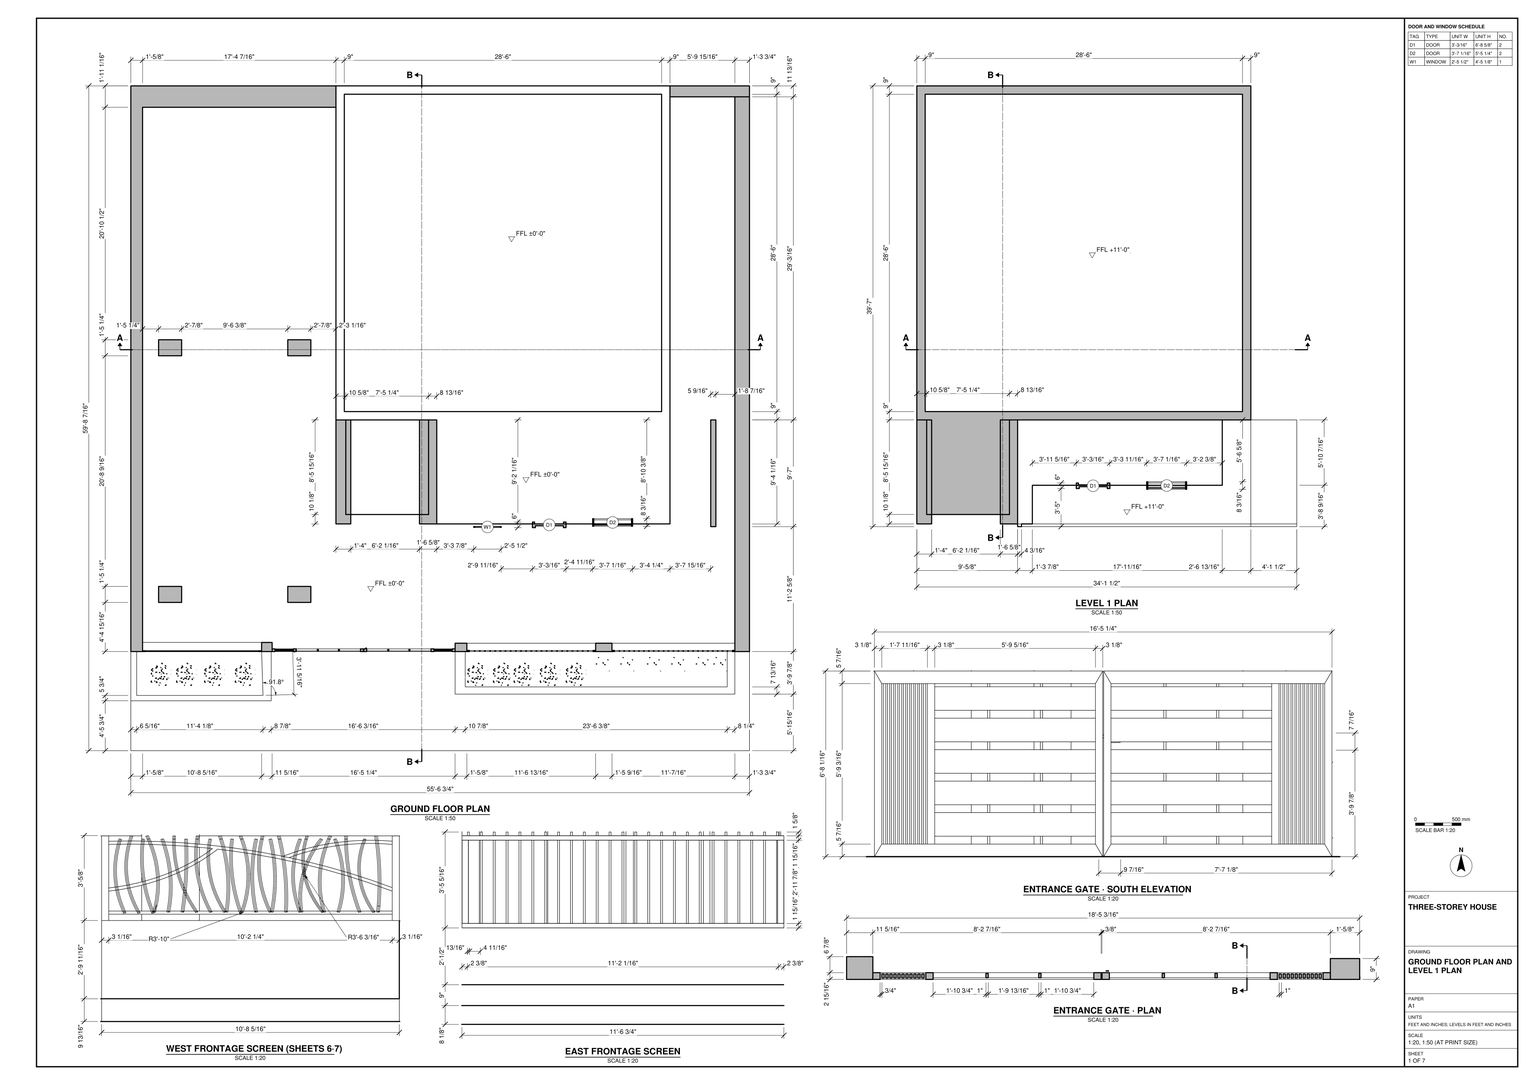
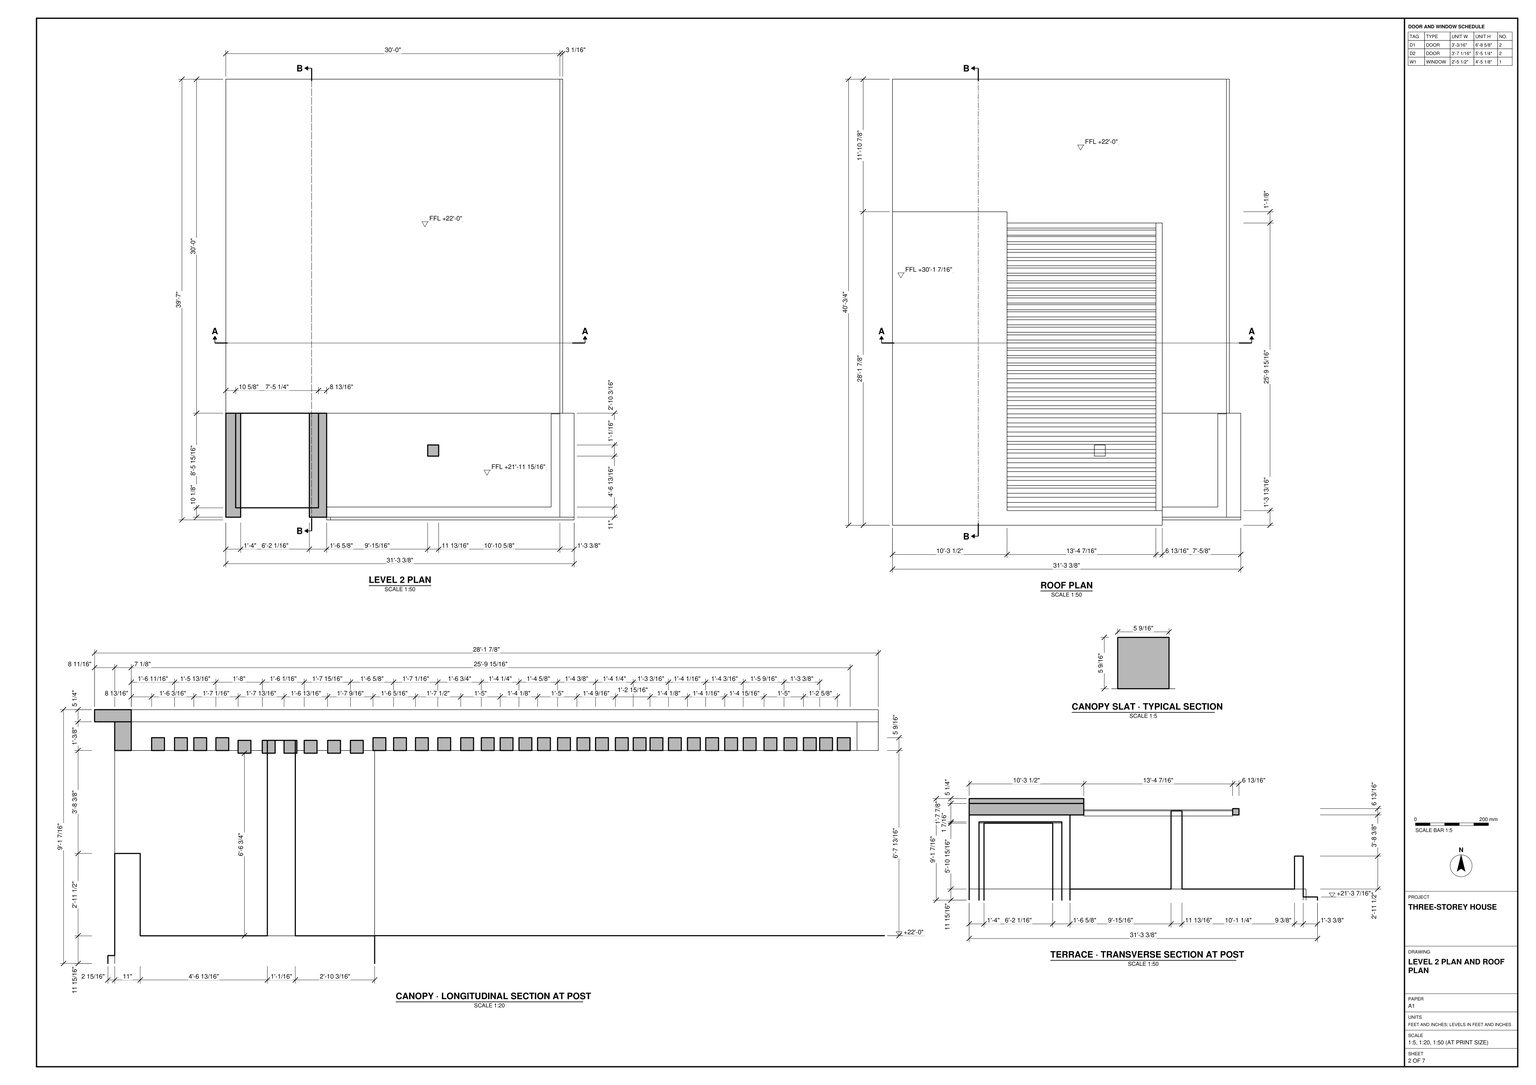
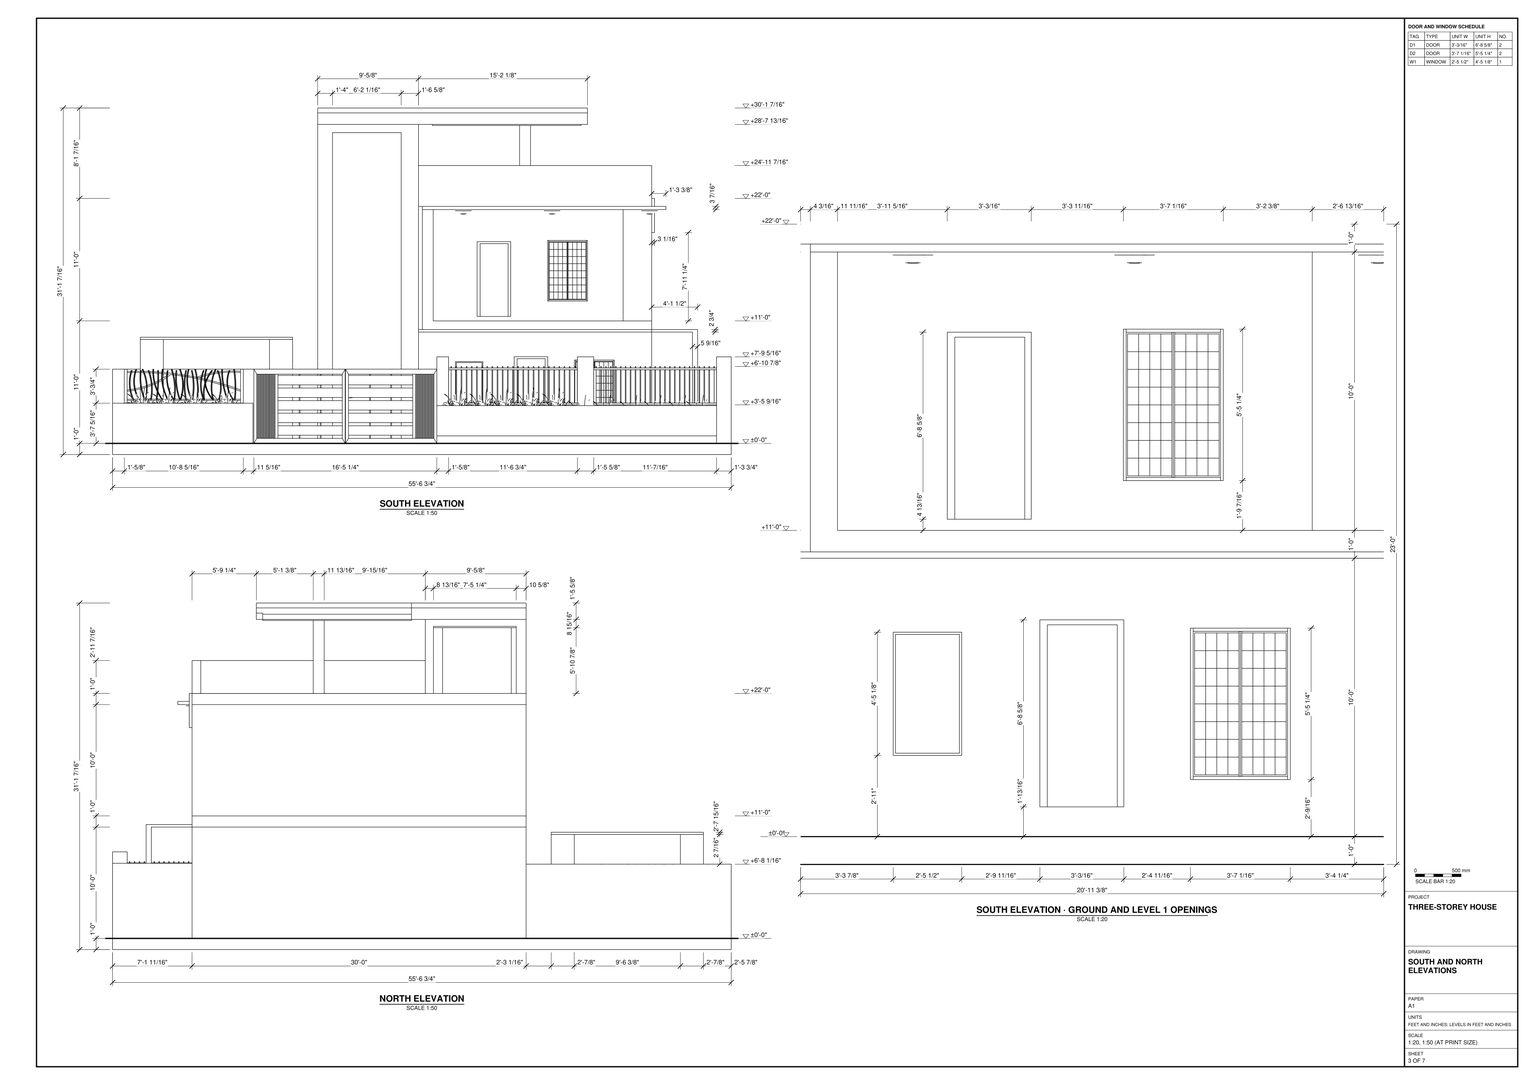
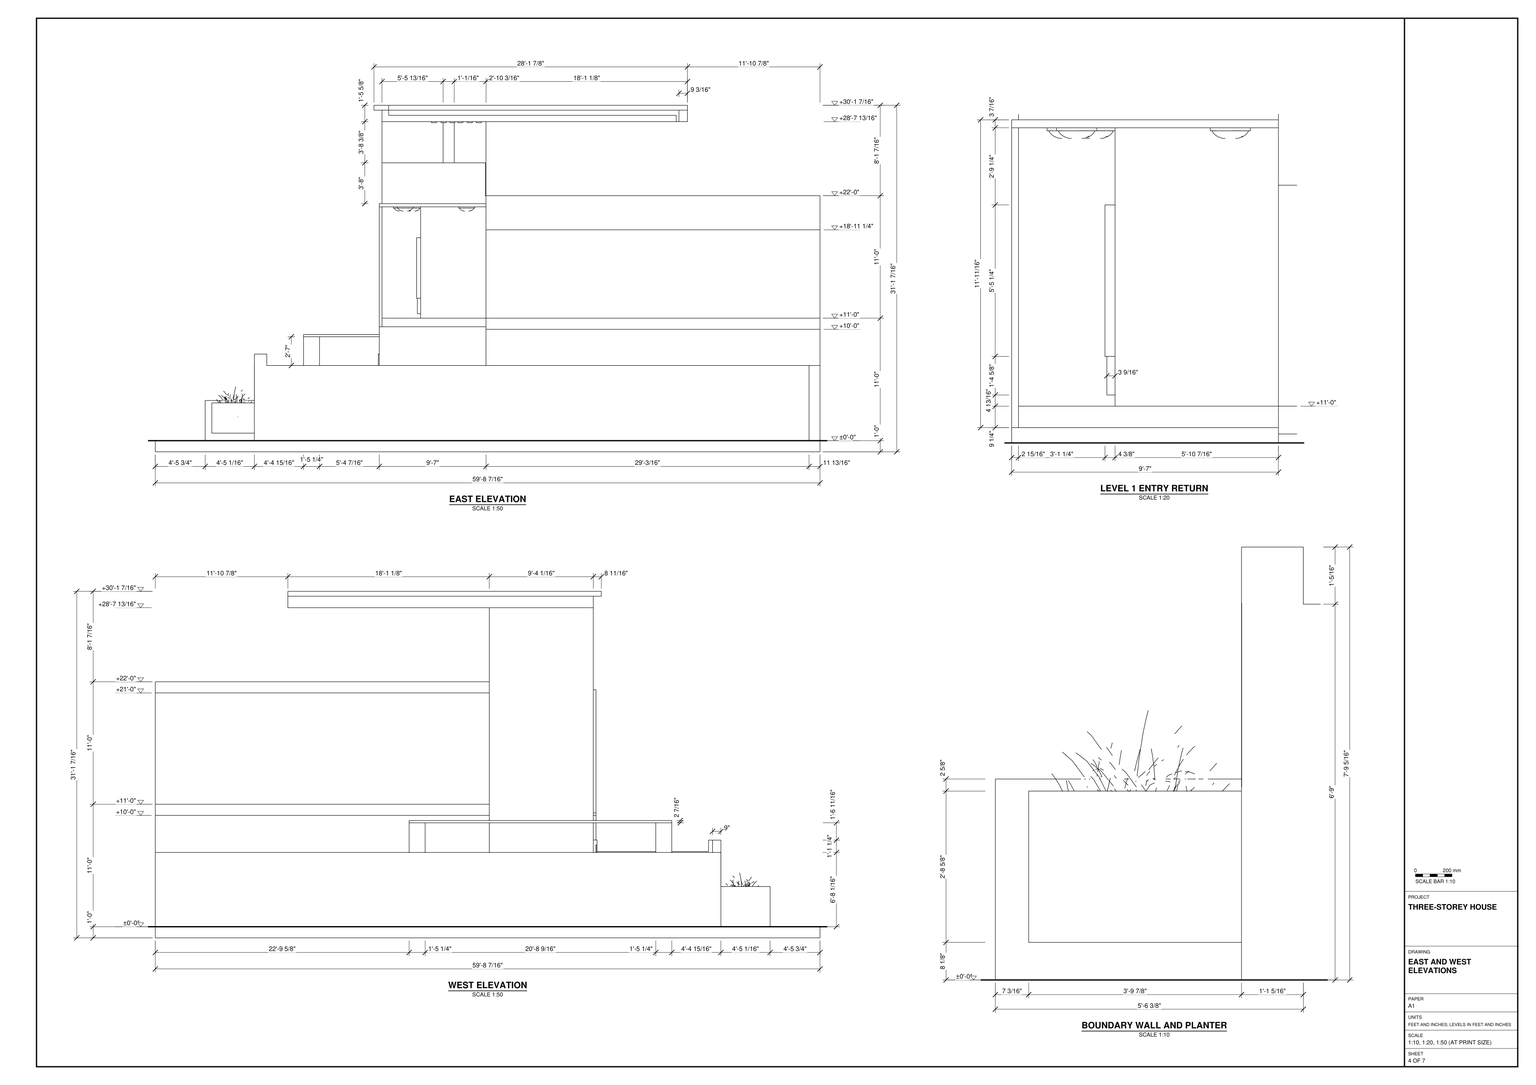
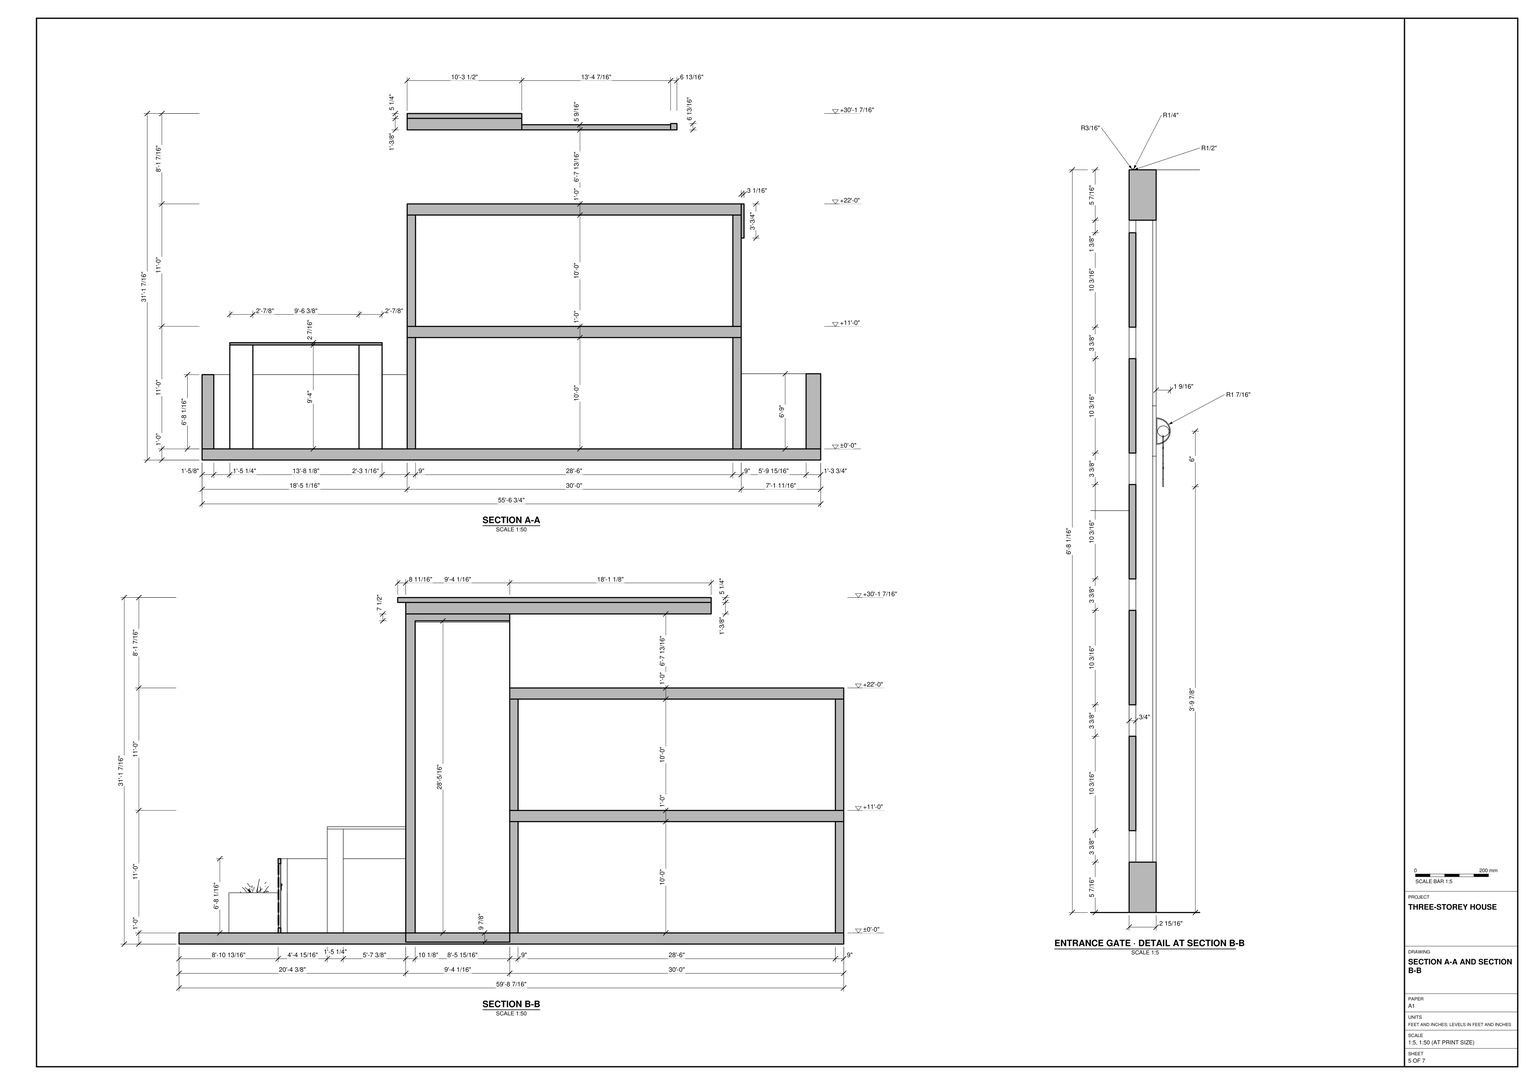
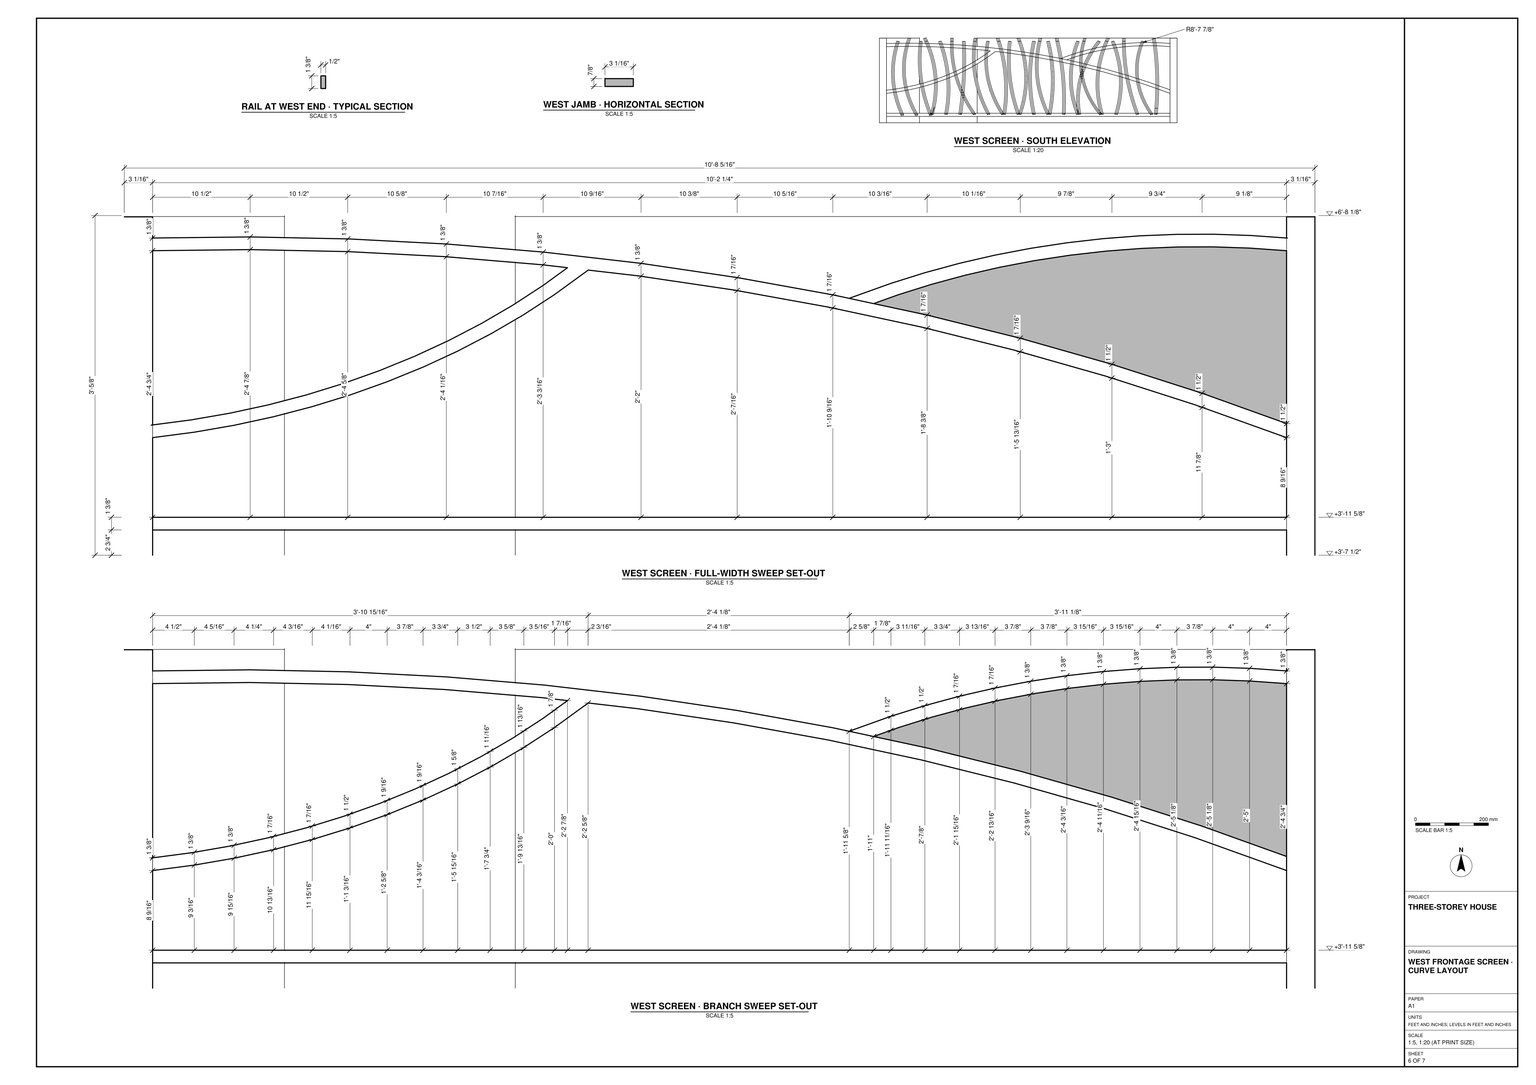
Work in feet and inches in SketchUp, using the plans, elevations, sections and details in task_files/diagram_01.pdf. Model the house and its enclosed site. The overall model measures 55'-6 3/4" east to west, 59'-8 7/16" north to south and 31'-1 7/16" high. Set the ground floor at ±0'-0", the next floor at +11'-0" and the terrace level at +22'-0".

Place the main block toward the rear of the site, leaving the forecourt between the house and the south entrance. Follow the wall thicknesses on the plans, including the 9" walls of the main block. Use the sections and elevations to set the slab edges, recesses and projections. Fit the doors, grilles and window in the south walls at the positions and heights shown. Above them, model the terrace parapet and the canopy, distinguishing its solid roof strip from the open span of parallel slats on posts.

Continue the site walls to the south frontage. Model the paired entrance gate, the curved-bar screen to its west, the vertical-bar screens to its east and the planting beds flanking the entrance. Decor and loose items, including plants, may be any suitable library components. Keep shell elements and individual furniture or joinery pieces in separate groups or components, and use components for repeated parts. Save one SketchUp model as output_files/three_storey_house_screened_frontage_and_terrace_canopy.skp.

# SketchUp Ruby script. Lengths in inches.
U = 1.inch
M = Sketchup.active_model
def pt(a) = Geom::Point3d.new(a.map { |v| v * U })
def face(e, loops, mat)
  f = e.add_face(loops[0].map { |a| pt(a) })
  loops[1..].each { |l| e.add_face(l.map { |a| pt(a) }).erase! }
  f.material = f.back_material = mat if mat
  f
end
# faces: each face lists its corners as indices into pts; further lists are holes
def faces(e, pts, list, mat = nil) = list.each { |f| face(e, (f[0].is_a?(Array) ? f : [f]).map { |l| l.map { |i| pts[i] } }, mat) }
# xy, xz, yz: faces in a plane at the given z, y or x. An outline is a flat list of corners, or four numbers for a rectangle; further outlines are holes
def ring(l) = l.size == 4 ? [[l[0], l[1]], [l[2], l[1]], [l[2], l[3]], [l[0], l[3]]] : l.each_slice(2).to_a
def flat(e, list, mat, &to3) = list.each { |f| face(e, (f[0].is_a?(Array) ? f : [f]).map { |l| ring(l).map { |u, v| to3.(u, v) } }, mat) }
def xy(e, z, list, mat = nil) = flat(e, list, mat) { |x, y| [x, y, z] }
def xz(e, y, list, mat = nil) = flat(e, list, mat) { |x, z| [x, y, z] }
def yz(e, x, list, mat = nil) = flat(e, list, mat) { |y, z| [x, y, z] }
def lines(e, pts, list) = list.each { |a, b| e.add_line(pt(pts[a]), pt(pts[b])) }
# prism: a flat outline (further loops are holes) pulled along v
def prism(e, loops, v, mat = nil)
  f = face(e, loops, mat); d = Geom::Vector3d.new(v.map { |x| x * U })
  f.pushpull(f.normal.samedirection?(d) ? d.length : -d.length)
end
def box(e, o, s, mat = nil) = prism(e, [[o, [o[0] + s[0], o[1], o[2]], [o[0] + s[0], o[1] + s[1], o[2]], [o[0], o[1] + s[1], o[2]]]], [0, 0, s[2]], mat)
def at(x, y, z, deg = 0) = Geom::Transformation.translation(pt([x, y, z])) * Geom::Transformation.rotation(ORIGIN, Z_AXIS, deg.degrees)
def axes(o, x, y, z) = Geom::Transformation.new([*x, 0, *y, 0, *z, 0, *pt(o).to_a, 1])
def part(name) = M.definitions.add(name)
# library, detail: a bought-in or finely detailed component or shape, given as its bounding box
def library(name, o, s) = part(name).tap { |d| box(d.entities, o, s) }
def detail(e, o, s) = box(e.add_group.entities, o, s)
def put(e, d, t, mat = nil) = e.add_instance(d, t).tap { |i| i.material = mat if mat }
def group(e, t, mat = nil) = e.add_group.tap { |g| g.transformation = t; g.material = mat if mat }.entities
root = M.entities
M.materials.add("Shane").color = [124, 51, 43]
M.materials.add("[Color M00]").color = [255, 255, 255]
M.materials.add("[Color M07]").color = [58, 58, 58]
M.materials.add("[Color M08]").color = [30, 30, 30]
M.materials.add("[Gray4]").color = [170, 170, 170]
M.materials.add("[Gray8]").color = [68, 68, 68]
M.materials.add("[Slate]").color = [102, 110, 108]
M.materials.add("[Translucent Glass Gray]3").color = [128, 128, 128]
M.materials["[Translucent Glass Gray]3"].alpha = 0.3
M.materials.add("[Translucent_Glass_Gray]").color = [128, 128, 128]
M.materials["[Translucent_Glass_Gray]"].alpha = 0.5
M.materials.add("[Wood Floor Light]").color = [204, 176, 127]
M.materials.add("[Wood Floor]").color = [155, 105, 61]
M.materials.add("[Wood_Cherry_Original]").color = [152, 86, 42]
c1 = part("door 15\#1")
xy(c1.entities,0,[[0,0,0,6,2.34,6,2.34,4,33.41,4,33.41,6,36.21,6,36.21,0,33.4,0,33.4,2,3.22,2,3.22,0]],"Shane")
xy(c1.entities,78.49,[[3.22,0,33.4,2]],"Shane")
xy(c1.entities,78.6875,[[2.34,4,33.41,6]],"Shane")
xy(c1.entities,80.63,[[0,0,36.21,6]],"Shane")
xz(c1.entities,0,[[0,0,3.22,0,3.22,78.49,33.4,78.49,33.4,0,36.21,0,36.21,80.63,0,80.63]],"Shane")
xz(c1.entities,2,[[3.22,0,33.4,78.49]],"Shane")
xz(c1.entities,4,[[2.34,0,33.41,78.6875]],"Shane")
xz(c1.entities,6,[[0,0,0,80.63,36.21,80.63,36.21,0,33.41,0,33.41,78.6875,2.34,78.6875,2.34,0]],"Shane")
yz(c1.entities,0,[[0,0,6,80.63]],"Shane")
yz(c1.entities,2.34,[[4,0,6,78.6875]],"Shane")
yz(c1.entities,3.22,[[0,0,2,78.49]],"Shane")
yz(c1.entities,33.4,[[0,0,2,78.49]],"Shane")
yz(c1.entities,33.41,[[4,0,6,78.6875]],"Shane")
yz(c1.entities,36.21,[[0,0,6,80.63]],"Shane")
c2 = part("glass door")
xy(c2.entities,0,[[0,-12,72,0]],"[Wood_Cherry_Original]")
xy(c2.entities,2,[[35,-10,36,-8],[36,-10,37,-8]],"[Gray4]")
xy(c2.entities,2,[[2,-10,35,-8],[37,-10,70,-8]],"[Gray8]")
xy(c2.entities,2,[[2,-12,70,-10],[2,-8,70,-2],[2,-2,70,0]],"[Wood_Cherry_Original]")
xy(c2.entities,94,[[35,-10,36,-8],[36,-10,37,-8]],"[Gray4]")
xy(c2.entities,94,[[2,-10,35,-8],[37,-10,70,-8]],"[Gray8]")
xy(c2.entities,94,[[2,-12,70,-10],[2,-8,70,0]],"[Wood_Cherry_Original]")
xy(c2.entities,96,[[0,-12,2,0],[2,-12,70,0],[70,-12,72,0]],"[Wood_Cherry_Original]")
xz(c2.entities,-12,[[0,0,2,96],[2,0,70,2],[70,0,72,96],[2,94,70,96]],"[Wood_Cherry_Original]")
xz(c2.entities,-10,[[3,3,11,14.25],[11,3,19,14.25],[19,3,27,14.25],[27,3,35,14.25],[37,3,45,14.25],
  [45,3,53,14.25],[53,3,61,14.25],[61,3,69,14.25],[3,14.25,11,25.5],[11,14.25,19,25.5],
  [19,14.25,27,25.5],[27,14.25,35,25.5],[37,14.25,45,25.5],[45,14.25,53,25.5],[53,14.25,61,25.5],
  [61,14.25,69,25.5],[3,25.5,11,36.75],[11,25.5,19,36.75],[19,25.5,27,36.75],[27,25.5,35,36.75],
  [37,25.5,45,36.75],[45,25.5,53,36.75],[53,25.5,61,36.75],[61,25.5,69,36.75],[3,36.75,11,48],
  [11,36.75,19,48],[19,36.75,27,48],[27,36.75,35,48],[37,36.75,45,48],[45,36.75,53,48],
  [53,36.75,61,48],[61,36.75,69,48],[3,48,11,59.25],[11,48,19,59.25],[19,48,27,59.25],
  [27,48,35,59.25],[37,48,45,59.25],[45,48,53,59.25],[53,48,61,59.25],[61,48,69,59.25],
  [3,59.25,11,70.5],[11,59.25,19,70.5],[19,59.25,27,70.5],[27,59.25,35,70.5],[37,59.25,45,70.5],
  [45,59.25,53,70.5],[53,59.25,61,70.5],[61,59.25,69,70.5],[3,70.5,11,81.75],[11,70.5,19,81.75],
  [19,70.5,27,81.75],[27,70.5,35,81.75],[37,70.5,45,81.75],[45,70.5,53,81.75],[53,70.5,61,81.75],
  [61,70.5,69,81.75],[3,81.75,11,93],[11,81.75,19,93],[19,81.75,27,93],[27,81.75,35,93],
  [37,81.75,45,93],[45,81.75,53,93],[53,81.75,61,93],[61,81.75,69,93]],"[Translucent_Glass_Gray]")
xz(c2.entities,-10,[[2,2,2,94,35,94,35,93,3,93,3,3,35,3,35,2],[35,2,36,94],[36,2,37,94],[37,2,37,3,69,3,69,93,37,93,37,94,70,94,70,2]],"[Wood_Cherry_Original]")
xz(c2.entities,0,[[0,0,72,0,72,96,70,96,70,2,2,2,2,96,0,96],[2,94,70,96]],"[Wood_Cherry_Original]")
yz(c2.entities,0,[[-12,0,0,96]],"[Wood_Cherry_Original]")
yz(c2.entities,2,[[-12,94,-10,96],[-10,94,-8,96],[-8,94,-2,96],[-2,94,0,96]])
yz(c2.entities,2,[[-10,2,-8,94]],"[Gray8]")
yz(c2.entities,2,[[-12,2,-10,94],[-8,2,-2,94],[-2,2,0,94]],"[Wood_Cherry_Original]")
yz(c2.entities,70,[[-12,94,-10,96],[-10,94,-8,96],[-8,94,-2,96],[-2,94,0,96]])
yz(c2.entities,70,[[-10,2,-8,94]],"[Gray8]")
yz(c2.entities,70,[[-12,2,-10,94],[-8,2,-2,94],[-2,2,0,94]],"[Wood_Cherry_Original]")
yz(c2.entities,72,[[-12,0,0,96]],"[Wood_Cherry_Original]")
c3 = part("WINDOW")
xy(c3.entities,0,[[0,0,59.06,1.97]],"[Color M07]")
xy(c3.entities,1.97,[[1.97,0,57.09,0.98],[1.97,0.98,57.09,1.97]],"[Color M07]")
xy(c3.entities,104.33,[[1.97,0,57.09,0.98],[1.97,0.98,57.09,1.97]],"[Color M07]")
xy(c3.entities,106.3,[[0,0,59.06,1.97]],"[Color M07]")
xz(c3.entities,0,[[[0,0,59.06,106.3],[1.97,1.97,57.09,104.33]]],"[Color M07]")
xz(c3.entities,0.98,[[1.97,1.97,57.09,104.33]],"[Translucent Glass Gray]3")
xz(c3.entities,1.97,[[[0,0,59.06,106.3],[1.97,1.97,57.09,104.33]]],"[Color M07]")
yz(c3.entities,0,[[0,0,1.97,106.3]],"[Color M07]")
yz(c3.entities,1.97,[[0,1.97,0.98,104.33],[0.98,1.97,1.97,104.33]],"[Color M07]")
yz(c3.entities,57.09,[[0,1.97,0.98,104.33],[0.98,1.97,1.97,104.33]],"[Color M07]")
yz(c3.entities,59.06,[[0,0,1.97,106.3]],"[Color M07]")
c4 = part("Group\#428")
prism(c4.entities,[[[0,1.97,0],[0,1.97,1.18],[0,0,1.18],[0,0,0]],[[0,1.92,1.13],[0,1.92,0.05],[0,0.05,0.05],[0,0.05,1.13]]],[98.43,0,0])
c5 = part("Group\#430")
xy(c5.entities,0,[[0.3,0,0.22,0.01,0.15,0.04,0.09,0.09,0.04,0.15,0.01,0.22,0,0.3,0.3,0.3],[0.3,0,0.3,0.3,0.59,0.3,0.58,0.22,0.55,0.15,0.5,0.09,0.44,0.04,0.37,0.01],[0,0.3,0.01,0.37,0.04,0.44,0.09,0.5,0.15,0.55,0.22,0.58,0.3,0.59,0.3,0.3],[0.3,0.3,0.3,0.59,0.37,0.58,0.44,0.55,0.5,0.5,0.55,0.44,0.58,0.37,0.59,0.3]])
xy(c5.entities,39.37,[[0.3,0,0.37,0.01,0.44,0.04,0.5,0.09,0.55,0.15,0.58,0.22,0.59,0.3,0.58,0.37,0.55,0.44,0.5,0.5,0.44,0.55,0.37,0.58,0.3,0.59,0.22,0.58,0.15,0.55,0.09,0.5,0.04,0.44,0.01,0.37,0,0.3,0.01,0.22,0.04,0.15,0.09,0.09,0.15,0.04,0.22,0.01]])
p = [[0.09,0.09,0],[0.15,0.04,0],[0.15,0.04,39.37],[0.09,0.09,39.37],[0.22,0.01,0],[0.22,0.01,39.37],
  [0.3,0,0],[0.3,0,39.37],[0.37,0.01,0],[0.37,0.01,39.37],[0.44,0.04,0],[0.44,0.04,39.37],
  [0.5,0.09,0],[0.5,0.09,39.37],[0.01,0.22,0],[0.04,0.15,0],[0.04,0.15,39.37],[0.01,0.22,39.37],
  [0.55,0.15,0],[0.55,0.15,39.37],[0.58,0.22,0],[0.58,0.22,39.37],[0,0.3,0],[0,0.3,39.37],
  [0.59,0.3,0],[0.59,0.3,39.37],[0.01,0.37,0],[0.01,0.37,39.37],[0.58,0.37,0],[0.58,0.37,39.37],
  [0.09,0.5,0],[0.04,0.44,0],[0.04,0.44,39.37],[0.09,0.5,39.37],[0.55,0.44,0],[0.5,0.5,0],
  [0.5,0.5,39.37],[0.55,0.44,39.37],[0.15,0.55,0],[0.15,0.55,39.37],[0.44,0.55,0],[0.44,0.55,39.37],
  [0.22,0.58,0],[0.22,0.58,39.37],[0.3,0.59,0],[0.3,0.59,39.37],[0.37,0.58,0],[0.37,0.58,39.37]]
faces(c5.entities,p,[[0,1,2,3],[1,4,5,2],[4,6,7,5],[6,8,9,7],[8,10,11,9],[10,12,13,11],[14,15,16,17],[15,0,3,16],
  [12,18,19,13],[18,20,21,19],[22,14,17,23],[20,24,25,21],[26,22,23,27],[24,28,29,25],[30,31,32,33],[31,26,27,32],
  [34,35,36,37],[28,34,37,29],[38,30,33,39],[35,40,41,36],[42,38,39,43],[44,42,43,45],[46,44,45,47],[40,46,47,41]])
c6 = part("Group\#429")
prism(c6.entities,[[[0.01,0.22,35.83],[0,0.3,35.83],[0.01,0.37,35.83],[0.04,0.44,35.83],[0.09,0.5,35.83],[0.15,0.55,35.83],[0.22,0.58,35.83],[0.3,0.59,35.83],[0.37,0.58,35.83],[0.44,0.55,35.83],[0.5,0.5,35.83],[0.55,0.44,35.83],[0.58,0.37,35.83],[0.59,0.3,35.83],[0.58,0.22,35.83],[0.55,0.15,35.83],[0.5,0.09,35.83],[0.44,0.04,35.83],[0.37,0.01,35.83],[0.3,0,35.83],[0.22,0.01,35.83],[0.15,0.04,35.83],[0.09,0.09,35.83],[0.04,0.15,35.83]]],[0,0,3.54])
c7 = part("Metal railing panel")
g1 = group(c7.entities,at(0,0,0))
put(g1,c4,axes([0,0,39.76],[1,0,0],[0,0,-1],[0,1,0]),"[Color M08]")
put(g1,c4,axes([0,0,1.97],[1,0,0],[0,0,-1],[0,1,0]),"[Color M08]")
put(g1,c4,axes([98.43,0,37.8],[0,0,-0.364],[-1,0,0],[0,1,0]),"[Color M08]")
put(g1,c4,axes([1.97,0,37.8],[0,0,-0.364],[-1,0,0],[0,1,0]),"[Color M08]")
g2 = group(c7.entities,at(1.67,0.3,1.97))
put(g2,c5,at(78.74,0,0),"[Color M08]")
put(g2,c5,at(90.55,0,0),"[Color M08]")
put(g2,c5,at(82.68,0,0),"[Color M08]")
put(g2,c5,at(86.61,0,0),"[Color M08]")
put(g2,c5,at(66.93,0,0),"[Color M08]")
put(g2,c5,at(11.8125,0,0),"[Color M08]")
put(g2,c5,at(15.75,0,0),"[Color M08]")
put(g2,c5,at(47.24,0,0),"[Color M08]")
put(g2,c5,at(59.06,0,0),"[Color M08]")
put(g2,c6,at(0,0,0),"[Color M08]")
put(g2,c5,at(39.37,0,0),"[Color M08]")
put(g2,c5,at(62.99,0,0),"[Color M08]")
put(g2,c5,at(55.12,0,0),"[Color M08]")
put(g2,c5,at(19.69,0,0),"[Color M08]")
put(g2,c5,at(35.43,0,0),"[Color M08]")
put(g2,c5,at(7.875,0,0),"[Color M08]")
put(g2,c5,at(23.62,0,0),"[Color M08]")
put(g2,c5,at(31.5,0,0),"[Color M08]")
put(g2,c5,at(43.31,0,0),"[Color M08]")
put(g2,c5,at(27.56,0,0),"[Color M08]")
put(g2,c5,at(3.9375,0,0),"[Color M08]")
put(g2,c5,at(51.18,0,0),"[Color M08]")
put(g2,c5,at(70.87,0,0),"[Color M08]")
put(g2,c5,at(74.8,0,0),"[Color M08]")
put(g2,c6,at(94.49,0,0),"[Color M08]")
c8 = library("Untitled",[133.32,-114.77,0],[197.24,2.41,46.46])
c9 = library("grille",[0,0,0],[82.68,1.97,31.62])
c10 = library("skatter_medium_grass_01_small_full",[-2.7,-2.61,-0.01],[5.25,5.67,5.05])
c11 = library("CM1021-ceilingfixture-VisaLighting.dwg",[51.34,51.34,0],[17.32,17.32,4.91])
c12 = part("CM1021")
put(c12.entities,c11,at(-570.38,72.59,247.09))
put(c12.entities,c11,at(-474.88,60.59,247.09))
put(c12.entities,c11,at(-369.81,130.94,247.09))
put(c12.entities,c11,at(-369.81,64.69,247.09))
c13 = part("Group\#24")
box(c13.entities,[0,0,0],[5.53,5.53,160.4375])
box(root,[29.88,159.78,112],[164.13,283.06,2.4375])
xy(root,-9.875,[[311.08,244.375,329.71,356.4375]])
xy(root,0,[[0,106.8125,0,716.4375,221.0625,716.4375,221.0625,693.37,12.62,693.37,12.62,106.8125],[12.62,106.8125,140.95,116.68],[140.95,106.8125,152.26,116.625],[349.51,106.8125,651.01,115.8125],[651.01,106.8125,666.75,704.65],
  [624.98,241.4375,630.5625,356.4375],[221.0625,244.375,221.0625,356.4375,231.67,356.4375,231.67,254.5,237.03,254.5,237.03,244.375],[[329.71,244.375,329.71,356.4375,221.0625,356.4375,221.0625,716.4375,581.0625,716.4375,581.0625,244.375],[230.0625,365.4375,572.0625,707.4375]],[231.67,254.5,237.03,356.4375],[237.03,254.5,320.92,356.4375],
  [230.0625,365.4375,572.0625,707.4375],[581.0625,704.65,666.75,716.4375]])
xy(root,8.1,[[349.51,60.9375,651.01,106.8125]])
xy(root,9.8125,[[6.31,59.51,6.31,106.8125,140.95,106.8125,142.43,59.51]])
xy(root,17.09,[[360.41,68.75,642.78,106.8125]])
xy(root,40.72,[[349.51,60.9375,651.01,60.9375,651.01,106.8125,642.78,106.8125,642.78,68.75,360.41,68.75,360.41,106.8125,349.51,106.8125]])
xy(root,41.5625,[[362.15,106.8125,500.98,115.8125],[518.54,106.8125,651.01,115.8125]])
xy(root,43.3125,[[0,53.75,0,106.8125,6.31,106.8125,6.31,59.51,142.43,59.51,140.95,106.8125,151.3125,106.8125,151.3125,53.75]])
xy(root,43.53,[[12.62,106.8125,140.95,116.68]])
xy(root,80.04,[[0,106.8125,12.62,106.8125,12.62,693.37,221.0625,693.37,221.0625,716.4375,0,716.4375],[140.95,106.8125,152.26,116.625]])
xy(root,81,[[651.01,120.13,666.75,704.65],[581.0625,704.65,666.75,716.4375]])
xy(root,93.3125,[[349.51,106.8125,362.15,115.8125],[500.98,106.8125,518.54,115.8125],[651.01,106.8125,666.75,120.13]])
xy(root,120,[[329.71,241.4375,581.0625,244.375],[329.71,244.375,581.0625,356.4375],[[221.0625,356.4375,581.0625,716.4375],[230.0625,365.4375,572.0625,707.4375]]])
xy(root,120,[[581.0625,241.4375,624.98,356.4375]],"[Wood Floor]")
xy(root,122.74,[[333.89,241.4375,581.0625,244.375]])
xy(root,122.74,[[581.0625,241.4375,630.5625,244.375],[581.0625,244.375,630.5625,356.4375]],"[Wood Floor]")
xy(root,132,[[[221.0625,356.4375,581.0625,716.4375],[230.0625,365.4375,572.0625,707.4375]],[230.0625,365.4375,572.0625,707.4375]])
xy(root,132,[[345.58,244.375,581.0625,244.375,581.0625,356.4375,550.27,356.4375,550.27,286,345.58,286]],"[Slate]")
xy(root,227.25,[[581.0625,356.4375,584.125,716.4375]])
xy(root,252,[[333.89,241.4375,333.89,244.375,345.58,244.375,345.58,286,550.27,286,550.27,356.4375,596.4375,356.4375,596.4375,241.4375],[[221.0625,356.4375,581.0625,716.4375],[230.0625,365.4375,572.0625,707.4375]]])
xy(root,255.44,[[329.71,241.4375,333.89,244.375],[333.89,241.4375,596.4375,244.375],[581.0625,244.375,596.4375,356.4375]])
xy(root,263.9375,[[[329.71,255.36,571.6875,255.36,571.6875,355.8,581.0625,355.8,581.0625,356.4375,329.71,356.4375],[438.65,310.18,450.46,322.24]]])
xy(root,264,[[581.0625,356.4375,584.125,716.4375]])
xy(root,299.4375,[[329.71,244.375,581.0625,244.375,581.0625,355.8,571.6875,355.8,571.6875,255.36,329.71,255.36]])
xy(root,334.875,[[237.03,244.375,311.08,356.4375]],"[Wood Floor]")
xy(root,336.3125,[[231.67,254.5,320.92,356.4375]])
xy(root,343.8125,[[221.0625,244.375,329.71,356.4375],[329.71,244.375,329.71,573.5625,344.58,573.5625,344.58,251.5,505.02,251.5,505.02,561.46,511.83,561.46,511.83,244.375],[221.0625,356.4375,329.71,573.5625]])
xy(root,348.1875,[[438.65,310.18,450.46,322.24]])
xy(root,350.625,[[505.02,251.5,511.83,561.46]])
xy(root,356.1875,[[221.0625,235.6875,511.83,244.375],[221.0625,244.375,221.0625,573.5625,344.58,573.5625,344.58,251.5,511.83,251.5,511.83,244.375]])
xy(root,361.4375,[[221.0625,235.6875,511.83,235.6875,511.83,251.5,344.58,251.5,344.58,573.5625,221.0625,573.5625]])
xz(root,53.75,[[0,0,151.3125,43.3125]])
xz(root,59.51,[[6.31,9.8125,142.43,43.3125]])
xz(root,60.9375,[[349.51,8.1,651.01,40.72]])
xz(root,68.75,[[360.41,17.09,642.78,40.72]])
xz(root,106.8125,[[0,0,12.62,0,12.62,9.8125,6.31,9.8125,6.31,43.3125,0,43.3125],[12.62,0,140.95,9.8125],[140.95,0,151.3125,43.3125],[151.3125,0,152.26,0,152.26,80.04,140.95,80.04,140.95,43.3125,151.3125,43.3125],[349.51,0,651.01,8.1],
  [651.01,0,666.75,93.3125],[6.31,9.8125,12.62,9.8125,12.62,80.04,0,80.04,0,43.3125,6.31,43.3125],[12.62,9.8125,140.95,43.53],[360.41,17.09,642.78,17.09,642.78,40.72,651.01,40.72,651.01,41.5625,518.54,41.5625,518.54,93.3125,500.98,93.3125,500.98,41.5625,362.15,41.5625,362.15,93.3125,349.51,93.3125,349.51,40.72,360.41,40.72]])
xz(root,115.8125,[[349.51,0,349.51,93.3125,362.15,93.3125,362.15,41.5625,500.98,41.5625,500.98,93.3125,518.54,93.3125,518.54,41.5625,651.01,41.5625,651.01,0]])
xz(root,116.625,[[140.95,0,152.26,80.04]])
xz(root,116.68,[[12.62,0,140.95,43.53]])
xz(root,120.13,[[651.01,81,666.75,93.3125]])
xz(root,235.6875,[[221.0625,356.1875,511.83,361.4375]])
xz(root,241.4375,[[329.71,120,581.0625,122.74],[329.71,122.74,333.89,255.44],[333.89,252,596.4375,255.44]])
xz(root,241.4375,[[624.98,0,630.5625,0,630.5625,122.74,581.0625,122.74,581.0625,120,624.98,120]],"[Wood Floor]")
xz(root,244.375,[[329.71,0,581.0625,120]])
xz(root,244.375,[[333.89,122.74,581.0625,122.74,581.0625,132,345.58,132,345.58,252,333.89,252],[329.71,255.44,581.0625,299.4375],[221.0625,343.8125,511.83,356.1875]],"[Slate]")
xz(root,244.375,[[311.08,-9.875,329.71,-9.875,329.71,343.8125,221.0625,343.8125,221.0625,0,237.03,0,237.03,334.875,311.08,334.875]],"[Wood Floor]")
xz(root,251.5,[[344.58,343.8125,344.58,356.1875,511.83,356.1875,511.83,350.625,505.02,350.625,505.02,343.8125],[344.58,356.1875,511.83,361.4375]])
xz(root,254.5,[[231.67,0,320.92,336.3125]],"[Slate]")
xz(root,255.36,[[329.71,263.9375,571.6875,299.4375]])
xz(root,286,[[345.58,132,550.27,252]],"[Wood Floor Light]")
xz(root,310.18,[[438.65,263.9375,450.46,348.1875]])
xz(root,322.24,[[438.65,263.9375,450.46,348.1875]])
xz(root,355.8,[[571.6875,263.9375,581.0625,299.4375]])
xz(root,356.4375,[[311.08,-9.875,329.71,0],[221.0625,0,231.67,120],[231.67,0,237.03,120],[237.03,0,311.08,120],[311.08,0,320.92,120],
  [320.92,0,329.71,120],[221.0625,120,231.67,132],[231.67,120,237.03,132],[237.03,120,311.08,132],[311.08,120,320.92,132],
  [320.92,120,329.71,132],[221.0625,132,231.67,252],[231.67,132,237.03,252],[311.08,132,320.92,252],[320.92,132,329.71,252],
  [329.71,132,345.58,252],[345.58,132,550.27,252],[581.0625,227.25,584.125,252],[221.0625,252,221.0625,343.8125,329.71,343.8125,329.71,252,320.92,252,320.92,336.3125,231.67,336.3125,231.67,252],[231.67,252,237.03,334.875],
  [237.03,252,311.08,334.875],[311.08,252,320.92,334.875],[329.71,252,581.0625,263.9375],[581.0625,252,584.125,255.44],[584.125,252,596.4375,255.44],
  [581.0625,255.44,584.125,264],[231.67,334.875,320.92,336.3125]])
xz(root,356.4375,[[550.27,132,581.0625,252]],"[Slate]")
xz(root,356.4375,[[624.98,0,624.98,120,329.71,120,329.71,132,581.0625,132,581.0625,122.74,630.5625,122.74,630.5625,0]],"[Wood Floor]")
xz(root,365.4375,[[230.0625,0,572.0625,120],[230.0625,132,572.0625,252]])
xz(root,561.46,[[505.02,343.8125,511.83,350.625]])
xz(root,573.5625,[[221.0625,343.8125,344.58,356.1875],[221.0625,356.1875,344.58,361.4375]])
xz(root,693.37,[[12.62,0,221.0625,80.04]])
xz(root,704.65,[[581.0625,0,651.01,81],[651.01,0,666.75,81]])
xz(root,707.4375,[[230.0625,0,572.0625,120],[230.0625,132,572.0625,252]])
xz(root,716.4375,[[0,0,221.0625,80.04],[221.0625,0,581.0625,120],[581.0625,0,666.75,81],[221.0625,132,581.0625,252],[581.0625,227.25,584.125,264]])
yz(root,0,[[53.75,0,106.8125,43.3125],[106.8125,0,716.4375,80.04]])
yz(root,6.31,[[59.51,9.8125,106.8125,43.3125]])
yz(root,12.62,[[106.8125,0,116.68,43.53],[116.68,0,693.37,0,693.37,80.04,106.8125,80.04,106.8125,43.53,116.68,43.53]])
yz(root,140.95,[[106.8125,0,116.625,43.53],[116.625,0,116.68,43.53],[106.8125,43.53,116.625,80.04]])
yz(root,151.3125,[[53.75,0,106.8125,43.3125]])
yz(root,152.26,[[106.8125,0,116.625,80.04]])
yz(root,221.0625,[[244.375,0,356.4375,343.8125],[356.4375,0,356.4375,120,716.4375,120,716.4375,80.04,693.37,80.04,693.37,0],[693.37,0,716.4375,80.04],[356.4375,132,716.4375,252],[244.375,343.8125,573.5625,356.1875],
  [235.6875,356.1875,573.5625,361.4375]])
yz(root,230.0625,[[365.4375,0,707.4375,120],[365.4375,132,707.4375,252]])
yz(root,231.67,[[254.5,0,356.4375,336.3125]])
yz(root,237.03,[[244.375,0,356.4375,334.875]],"[Wood Floor]")
yz(root,311.08,[[244.375,-9.875,356.4375,334.875]],"[Wood Floor]")
yz(root,320.92,[[254.5,0,356.4375,336.3125]])
yz(root,329.71,[[244.375,-9.875,356.4375,0],[244.375,0,356.4375,120],[241.4375,120,244.375,122.74],[244.375,120,356.4375,120,356.4375,263.9375,255.36,263.9375,255.36,299.4375,244.375,299.4375],[241.4375,122.74,244.375,255.44]])
yz(root,329.71,[[255.36,263.9375,356.4375,263.9375,356.4375,343.8125,244.375,343.8125,244.375,299.4375,255.36,299.4375]],"[Wood Floor]")
yz(root,333.89,[[241.4375,122.74,244.375,252],[241.4375,252,244.375,255.44]])
yz(root,344.58,[[251.5,343.8125,564.41,356.1875],[564.41,343.8125,573.5625,356.1875],[251.5,356.1875,573.5625,361.4375]])
yz(root,345.58,[[244.375,132,286,252]],"[Slate]")
yz(root,349.51,[[106.8125,0,106.8125,8.1,60.9375,8.1,60.9375,40.72,106.8125,40.72,106.8125,93.3125,115.8125,93.3125,115.8125,0]])
yz(root,360.41,[[68.75,17.09,106.8125,40.72]])
yz(root,362.15,[[106.8125,41.5625,115.8125,93.3125]])
yz(root,438.65,[[310.18,263.9375,322.24,348.1875]])
yz(root,450.46,[[310.18,263.9375,322.24,348.1875]])
yz(root,500.98,[[106.8125,41.5625,115.8125,93.3125]])
yz(root,505.02,[[251.5,343.8125,561.46,350.625]])
yz(root,511.83,[[235.6875,356.1875,251.5,361.4375]])
yz(root,511.83,[[244.375,343.8125,561.46,343.8125,561.46,350.625,251.5,350.625,251.5,356.1875,244.375,356.1875]],"[Slate]")
yz(root,518.54,[[106.8125,41.5625,115.8125,93.3125]])
yz(root,550.27,[[286,132,356.4375,252]],"[Wood Floor Light]")
yz(root,571.6875,[[255.36,263.9375,355.8,299.4375]])
yz(root,572.0625,[[365.4375,0,707.4375,120],[365.4375,132,707.4375,252]])
yz(root,581.0625,[[244.375,0,704.65,0,704.65,81,716.4375,81,716.4375,120,244.375,120],[704.65,0,716.4375,81],[356.4375,132,716.4375,227.25],[356.4375,227.25,716.4375,252],[356.4375,252,716.4375,264]])
yz(root,581.0625,[[244.375,122.74,356.4375,132],[244.375,255.44,356.4375,255.44,356.4375,263.9375,355.8,263.9375,355.8,299.4375,244.375,299.4375]],"[Slate]")
yz(root,584.125,[[356.4375,227.25,716.4375,264]])
yz(root,596.4375,[[241.4375,252,356.4375,255.44]])
yz(root,624.98,[[241.4375,0,356.4375,120]],"[Wood Floor]")
yz(root,630.5625,[[241.4375,0,356.4375,122.74]],"[Wood Floor]")
yz(root,642.78,[[68.75,17.09,106.8125,40.72]])
yz(root,651.01,[[106.8125,0,115.8125,41.5625],[115.8125,0,115.8125,41.5625,106.8125,41.5625,106.8125,93.3125,120.13,93.3125,120.13,81,704.65,81,704.65,0],[60.9375,8.1,106.8125,40.72]])
yz(root,666.75,[[106.8125,0,704.65,0,704.65,81,120.13,81,120.13,93.3125,106.8125,93.3125],[704.65,0,716.4375,81]])
p = [[142.43,59.51,9.8125],[140.95,106.8125,9.8125],[140.95,106.8125,43.3125],[142.43,59.51,43.3125],[344.58,251.5,356.1875],[301.14,251.5,356.1875]]
faces(root,p,[[0,1,2,3]])
lines(root,p,[[4,5]])
put(root,c1,at(392.92,282.47,136.8125))
put(root,c2,axes([468.83,289.8125,153.46],[0.5984,0,0],[0,0.68,0],[0,0,0.68]))
put(root,c1,at(432.82,240.375,12.82))
put(root,c2,axes([497.74,250.03,24.58],[0.5984,0,0],[0,0.68,0],[0,0,0.68]))
put(root,c3,axes([369.6,240.625,34.97],[0.5,0,0],[0,0.5,0],[0,0,0.5]))
put(root,c7,axes([362.15,106.8125,41.5625],[1.41,0,0],[0,1,0],[0,0,1]))
put(root,c7,axes([518.54,106.8125,41.5625],[1.34581,0,0],[0,1,0],[0,0,1]))
put(root,c8,axes([18.94,319.14,0],[1,0,0],[0,1.85,0],[0,0,1.7228]))
put(root,c9,axes([12.62,106.8125,43.53],[1.55219,0,0],[0,0.43,0],[0,0,1.1579]))
put(root,c10,axes([373.25,82.5,23.05],[6.5296,0,0],[0,6.5296,0],[0,0,7.33486]))
put(root,c10,axes([400.88,82.5,23.05],[6.5296,0,0],[0,6.5296,0],[0,0,7.33486]))
put(root,c10,axes([423.13,82.5,23.05],[6.5296,0,0],[0,6.5296,0],[0,0,7.33486]))
put(root,c10,axes([451.31,82.5,23.05],[6.5296,0,0],[0,6.5296,0],[0,0,7.33486]))
put(root,c10,axes([479.31,82.5,23.05],[6.5296,0,0],[0,6.5296,0],[0,0,7.33486]))
put(root,c10,axes([507.43,90,14.98],[6.5296,0,0],[0,6.5296,0],[0,0,7.33486]))
put(root,c10,axes([533.85,90,14.98],[6.5296,0,0],[0,6.5296,0],[0,0,7.33486]))
put(root,c10,axes([562.54,90,14.98],[6.5296,0,0],[0,6.5296,0],[0,0,7.33486]))
put(root,c10,axes([588.72,90,14.98],[6.5296,0,0],[0,6.5296,0],[0,0,7.33486]))
put(root,c10,axes([615.16,90,14.98],[6.5296,0,0],[0,6.5296,0],[0,0,7.33486]))
put(root,c10,axes([634.16,90,14.98],[6.5296,0,0],[0,6.5296,0],[0,0,7.33486]))
put(root,c10,axes([32,82.5,23.05],[6.5296,0,0],[0,6.5296,0],[0,0,7.33486]))
put(root,c10,axes([59.38,82.5,23.05],[6.5296,0,0],[0,6.5296,0],[0,0,7.33486]))
put(root,c10,axes([89.56,82.5,23.05],[6.5296,0,0],[0,6.5296,0],[0,0,7.33486]))
put(root,c10,axes([122.69,82.5,23.05],[6.5296,0,0],[0,6.5296,0],[0,0,7.33486]))
put(root,c12,at(888.52,144.75,0))
g3 = group(root,at(221.0625,716.4375,120))
box(g3,[0,-360,0],[360,360,12])
put(root,c13,axes([344.58,260.29,343.8125],[0,1,0],[0,0,1],[1,0,0]))
g4 = group(root,at(221.0625,716.4375,-12))
xy(g4,0,[[-221.0625,-716.4375,445.6875,0]])
xy(g4,12,[[-221.0625,-716.4375,445.6875,0]],"[Color M00]")
xz(g4,-716.4375,[[-221.0625,0,445.6875,12]])
xz(g4,0,[[-221.0625,0,445.6875,12]])
yz(g4,-221.0625,[[-716.4375,0,0,12]])
yz(g4,445.6875,[[-716.4375,0,0,12]])
g5 = group(root,at(221.0625,716.4375,252))
box(g5,[0,-360,0],[360,360,12])
put(root,c13,axes([344.58,270.16,343.8125],[0,1,0],[0,0,1],[1,0,0]))
put(root,c13,axes([344.58,278.48,343.8125],[0,1,0],[0,0,1],[1,0,0]))
put(root,c13,axes([344.58,288,343.8125],[0,1,0],[0,0,1],[1,0,0]))
put(root,c13,axes([344.58,297.5625,342.66],[0,1,0],[0,0,1],[1,0,0]))
put(root,c13,axes([344.58,308,342.66],[0,1,0],[0,0,1],[1,0,0]))
put(root,c13,axes([344.58,317.375,342.66],[0,1,0],[0,0,1],[1,0,0]))
put(root,c13,axes([344.58,326.0625,342.66],[0,1,0],[0,0,1],[1,0,0]))
put(root,c13,axes([344.58,336.1875,342.66],[0,1,0],[0,0,1],[1,0,0]))
put(root,c13,axes([344.58,346,342.66],[0,1,0],[0,0,1],[1,0,0]))
put(root,c13,axes([344.58,355.74,343.8125],[0,1,0],[0,0,1],[1,0,0]))
put(root,c13,axes([344.58,364.61,343.8125],[0,1,0],[0,0,1],[1,0,0]))
put(root,c13,axes([344.58,374.05,343.8125],[0,1,0],[0,0,1],[1,0,0]))
put(root,c13,axes([344.58,383.67,343.8125],[0,1,0],[0,0,1],[1,0,0]))
put(root,c13,axes([344.58,393.55,343.8125],[0,1,0],[0,0,1],[1,0,0]))
put(root,c13,axes([344.58,402.42,343.8125],[0,1,0],[0,0,1],[1,0,0]))
put(root,c13,axes([344.58,410.55,343.8125],[0,1,0],[0,0,1],[1,0,0]))
put(root,c13,axes([344.58,418.67,343.8125],[0,1,0],[0,0,1],[1,0,0]))
put(root,c13,axes([344.58,426.67,343.8125],[0,1,0],[0,0,1],[1,0,0]))
put(root,c13,axes([344.58,435.3,343.8125],[0,1,0],[0,0,1],[1,0,0]))
put(root,c13,axes([344.58,443.67,343.8125],[0,1,0],[0,0,1],[1,0,0]))
put(root,c13,axes([344.58,451.67,343.8125],[0,1,0],[0,0,1],[1,0,0]))
put(root,c13,axes([344.58,460.24,343.8125],[0,1,0],[0,0,1],[1,0,0]))
put(root,c13,axes([344.58,467.92,343.8125],[0,1,0],[0,0,1],[1,0,0]))
put(root,c13,axes([344.58,475.17,343.8125],[0,1,0],[0,0,1],[1,0,0]))
put(root,c13,axes([344.58,483.11,343.8125],[0,1,0],[0,0,1],[1,0,0]))
put(root,c13,axes([344.58,491.3,343.8125],[0,1,0],[0,0,1],[1,0,0]))
put(root,c13,axes([344.58,499.17,343.8125],[0,1,0],[0,0,1],[1,0,0]))
put(root,c13,axes([344.58,507.36,343.8125],[0,1,0],[0,0,1],[1,0,0]))
put(root,c13,axes([344.58,515.36,343.8125],[0,1,0],[0,0,1],[1,0,0]))
put(root,c13,axes([344.58,524.3,343.8125],[0,1,0],[0,0,1],[1,0,0]))
put(root,c13,axes([344.58,532.92,343.8125],[0,1,0],[0,0,1],[1,0,0]))
put(root,c13,axes([344.58,541.3,343.8125],[0,1,0],[0,0,1],[1,0,0]))
put(root,c13,axes([344.58,548.3,343.8125],[0,1,0],[0,0,1],[1,0,0]))
put(root,c13,axes([344.58,555.92,343.8125],[0,1,0],[0,0,1],[1,0,0]))
g6 = group(root,at(29.88,159.78,0))
box(g6,[0,0,0],[24.875,17.25,112])
g7 = group(root,at(169.13,159.78,0))
box(g7,[0,0,0],[24.875,17.25,112])
g8 = group(root,at(29.88,425.59,0))
box(g8,[0,0,0],[24.875,17.25,112])
g9 = group(root,at(169.13,425.59,0))
box(g9,[0,0,0],[24.875,17.25,112])
